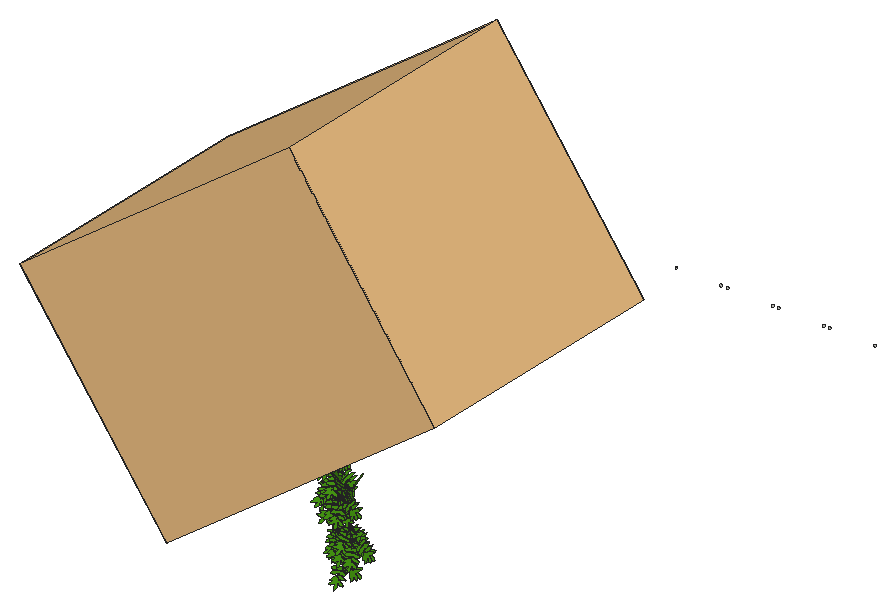
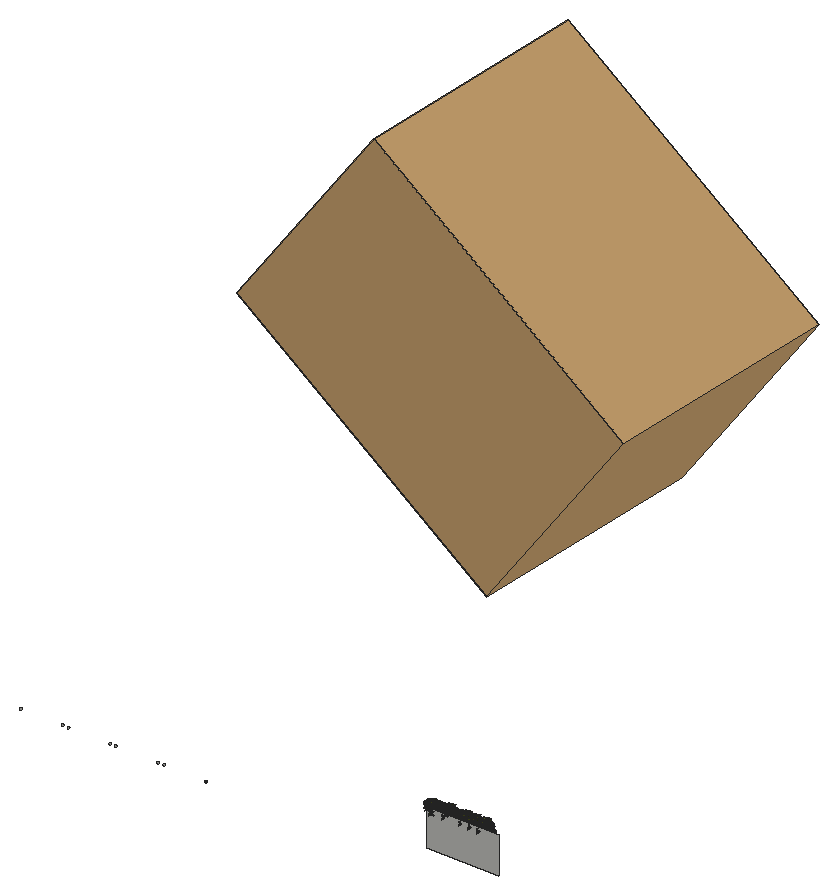
# SketchUp Ruby script. Lengths in inches.
U = 1.inch
M = Sketchup.active_model
def pt(a) = Geom::Point3d.new(a.map { |v| v * U })
def face(e, loops, mat)
  f = e.add_face(loops[0].map { |a| pt(a) })
  loops[1..].each { |l| e.add_face(l.map { |a| pt(a) }).erase! }
  f.material = f.back_material = mat if mat
  f
end
# faces: each face lists its corners as indices into pts; further lists are holes
def faces(e, pts, list, mat = nil) = list.each { |f| face(e, (f[0].is_a?(Array) ? f : [f]).map { |l| l.map { |i| pts[i] } }, mat) }
# xy, xz, yz: faces in a plane at the given z, y or x. An outline is a flat list of corners, or four numbers for a rectangle; further outlines are holes
def ring(l) = l.size == 4 ? [[l[0], l[1]], [l[2], l[1]], [l[2], l[3]], [l[0], l[3]]] : l.each_slice(2).to_a
def flat(e, list, mat, &to3) = list.each { |f| face(e, (f[0].is_a?(Array) ? f : [f]).map { |l| ring(l).map { |u, v| to3.(u, v) } }, mat) }
def xy(e, z, list, mat = nil) = flat(e, list, mat) { |x, y| [x, y, z] }
def xz(e, y, list, mat = nil) = flat(e, list, mat) { |x, z| [x, y, z] }
def yz(e, x, list, mat = nil) = flat(e, list, mat) { |y, z| [x, y, z] }
def lines(e, pts, list) = list.each { |a, b| e.add_line(pt(pts[a]), pt(pts[b])) }
# prism: a flat outline (further loops are holes) pulled along v
def prism(e, loops, v, mat = nil)
  f = face(e, loops, mat); d = Geom::Vector3d.new(v.map { |x| x * U })
  f.pushpull(f.normal.samedirection?(d) ? d.length : -d.length)
end
def box(e, o, s, mat = nil) = prism(e, [[o, [o[0] + s[0], o[1], o[2]], [o[0] + s[0], o[1] + s[1], o[2]], [o[0], o[1] + s[1], o[2]]]], [0, 0, s[2]], mat)
def at(x, y, z, deg = 0) = Geom::Transformation.translation(pt([x, y, z])) * Geom::Transformation.rotation(ORIGIN, Z_AXIS, deg.degrees)
def axes(o, x, y, z) = Geom::Transformation.new([*x, 0, *y, 0, *z, 0, *pt(o).to_a, 1])
def part(name) = M.definitions.add(name)
# library, detail: a bought-in or finely detailed component or shape, given as its bounding box
def library(name, o, s) = part(name).tap { |d| box(d.entities, o, s) }
def detail(e, o, s) = box(e.add_group.entities, o, s)
def put(e, d, t, mat = nil) = e.add_instance(d, t).tap { |i| i.material = mat if mat }
def group(e, t, mat = nil) = e.add_group.tap { |g| g.transformation = t; g.material = mat if mat }.entities
root = M.entities
M.materials.add("asdfasdfasdfasdf").color = [186, 198, 91]
M.materials.add("hojas").color = [70, 150, 19]
M.materials.add("leaf1_smaller_cleanasdfasfasdfas").color = [88, 95, 33]
M.materials.add("leaf2_smaller_cleansadfasdfasdfasd").color = [55, 66, 19]
c1 = part("rama-acacia")
p = [[-13.53,0.69,-1.07],[-13.38,0.86,-0.98],[-13.61,0.85,-1.06],[-14.07,0.85,-1.21],[-15.17,0.86,-1.58],[-15.95,0.92,-1.83],
  [-16.01,1,-1.83],[-16.01,1.17,-1.78],[-16.07,1.93,-1.6],[-16.4,2.73,-1.5],[-16.65,3.06,-1.5],[-17.13,4.01,-1.41],
  [-17.78,4.7,-1.44],[-18.28,5.07,-1.51],[-18.57,5.18,-1.58],[-18.91,5.47,-1.62],[-19.07,5.48,-1.67],[-19.35,5.61,-1.73],
  [-19.51,5.64,-1.78],[-19.38,5.57,-1.75],[-19.33,5.5,-1.75],[-19.31,5.23,-1.82],[-19.38,5.08,-1.89],[-19.41,4.84,-1.96],
  [-19.36,4.59,-2.01],[-19.43,4.55,-2.04],[-19.36,4.15,-2.125],[-19.21,3.7,-2.19],[-18.875,3.1,-2.24],[-18.61,2.78,-2.24],
  [-17.83,2.19,-2.13],[-17.4375,1.85,-2.09],[-17.04,1.49,-2.05],[-16.61,1.24,-1.97],[-16.17,1.0625,-1.87],[-16.06,0.95,-1.86],
  [-16.06,0.91,-1.87],[-16.32,0.9,-1.96],[-16.7,0.88,-2.1],[-17.05,0.91,-2.21],[-17.61,1.15,-2.33],[-18.06,1.29,-2.45],
  [-18.88,1.53,-2.67],[-20.25,1.46,-3.15],[-20.59,1.49,-3.26],[-20.79,1.37,-3.36],[-21.08,1.2,-3.5],[-21.28,1.22,-3.5625],
  [-21.48,0.94,-3.71],[-21.79,0.5,-3.93],[-22.02,0.17,-4.1],[-22.11,0.05,-4.16],[-22.21,-0.02,-4.21],[-22.375,-0.05,-4.28],
  [-22.375,-0.07,-4.28],[-22.18,-0.09,-4.22],[-22.11,-0.07,-4.19],[-21.78,-0.1,-4.09],[-21.6,-0.18,-4.05],[-21.52,-0.27,-4.04],
  [-21.33,-0.33,-4],[-20.94,-0.54,-3.92],[-20.6875,-0.63,-3.86],[-20.54,-0.68,-3.82],[-20.42,-0.67,-3.78],[-20.09,-0.46,-3.61],
  [-19.8,-0.24,-3.45],[-19.21,-0.02,-3.19],[-18.48,0.08,-2.92],[-17.72,0.38,-2.58],[-17.4,0.5,-2.4375],[-16.93,0.75,-2.21],
  [-16.78,0.8,-2.15],[-16.1,0.83,-1.91],[-16.0625,0.81,-1.9],[-16.08,0.77,-1.91],[-16.27,0.72,-1.99],[-16.88,0.39,-2.29],
  [-17.1875,0.15,-2.46],[-17.27,0.02,-2.52],[-17.94,-0.52,-2.89],[-17.94,-0.59,-2.91],[-18.08,-0.68,-2.99],[-18.13,-0.86,-3.05],
  [-18.56,-1.55,-3.38],[-18.71,-2.11,-3.58],[-18.79,-2.61,-3.74],[-18.86,-2.84,-3.83],[-18.87,-3.07,-3.89],[-18.84,-3.22,-3.92],
  [-18.8,-3.26,-3.92],[-18.76,-3.47,-3.96],[-18.76,-3.6,-4],[-18.67,-3.8,-4.02],[-18.61,-3.92,-4.04],[-18.58,-4.11,-4.07],
  [-18.53,-4.18,-4.08],[-18.58,-4.35,-4.14],[-18.65,-4.43,-4.18],[-18.72,-4.51,-4.23],[-18.8125,-4.51,-4.26],[-18.8125,-4.53,-4.26],
  [-18.72,-4.54,-4.24],[-18.66,-4.49,-4.21],[-18.58,-4.43,-4.16],[-18.35,-4.23,-4.03],[-18.32,-4.17,-4],[-18.22,-4.125,-3.95],
  [-18.1,-4,-3.88],[-17.79,-3.72,-3.7],[-17.68,-3.51,-3.61],[-17.32,-3.13,-3.38],[-17.24,-2.94,-3.31],[-16.78,-2.12,-2.93],
  [-16.48,-1.78,-2.73],[-16.3,-1.28,-2.54],[-16.05,-0.75,-2.3125],[-15.89,-0.2,-2.11],[-15.89,0.39,-1.95],[-15.96,0.79,-1.87],
  [-15.91,0.82,-1.84],[-15.27,0.8,-1.63],[-14.18,0.76,-1.27],[-13.78,0.73,-1.15],[-13.78,0.67,-1.16],[-14.23,0.54,-1.35],
  [-14.65,0.33,-1.55],[-14.97,0.02,-1.74],[-15.25,-0.36,-1.9375],[-15.57,-0.72,-2.14],[-15.96,-1.64,-2.52],[-16.2,-2.51,-2.84],
  [-16.2,-3.12,-3],[-16.14,-3.41,-3.06],[-16.1,-3.75,-3.14],[-16.1,-4.09,-3.23],[-16.2,-4.25,-3.3],[-16.2,-4.28,-3.3125],
  [-16.08,-4.19,-3.24],[-15.98,-4.08,-3.18],[-15.96,-3.94,-3.14],[-15.96,-3.8125,-3.1],[-15.9,-3.72,-3.06],[-15.68,-3.55,-2.9375],
  [-15.51,-3.49,-2.86],[-15.3,-3.33,-2.75],[-15.23,-3.17,-2.68],[-15.01,-3.03,-2.57],[-14.875,-2.83,-2.47],[-14.6,-2.59,-2.3125],
  [-14.4,-2.27,-2.16],[-14.12,-1.6,-1.89],[-13.91,-1.1,-1.68],[-13.67,-0.83,-1.53],[-13.53,-0.45,-1.38],[-13.53,0.67,-1.08],
  [-12.41,6.01,0.65],[-12.44,6.14,0.68],[-12.41,6.29,0.73],[-12.43,6.29,0.73],[-12.44,6.26,0.72],[-12.47,6.15,0.68],
  [-12.49,6.07,0.66],[-12.57,5.75,0.55],[-12.67,5.36,0.43],[-12.79,4.875,0.28],[-12.83,4.52,0.18],[-12.83,3.99,0.04],
  [-12.73,3.11,-0.18],[-12.58,2.52,-0.3125],[-12.3,1.97,-0.41],[-11.88,1.51,-0.46],[-11.37,1.0625,-0.48],[-10.75,0.75,-0.45],
  [-10.75,0.68,-0.47],[-12.55,0.7,-0.79],[-13.21,0.79,-0.89],[-13.2,0.67,-0.92],[-12.56,0.62,-0.82],[-11.15,0.56,-0.58],
  [-10.79,0.54,-0.52],[-10.72,0.52,-0.51],[-10.72,0.5,-0.52],[-10.87,0.47,-0.55],[-11.14,0.41,-0.62],[-11.39,0.27,-0.7],
  [-11.625,-0.01,-0.82],[-11.8,-0.43,-0.96],[-11.83,-0.57,-1],[-12.02,-1.08,-1.17],[-12.1,-1.39,-1.27],[-12.17,-1.95,-1.4375],
  [-12.17,-2.77,-1.65],[-12.09,-3.59,-1.86],[-11.86,-4.26,-2],[-11.8125,-4.4,-2.03],[-11.84,-4.49,-2.05],[-11.91,-4.6,-2.1],
  [-11.97,-4.65,-2.12],[-11.98,-4.67,-2.13],[-11.92,-4.65,-2.11],[-11.84,-4.59,-2.08],[-11.77,-4.52,-2.05],[-11.74,-4.47,-2.03],
  [-11.37,-4.3125,-1.92],[-10.95,-4.0625,-1.78],[-10.82,-3.89,-1.71],[-10.64,-3.57,-1.59],[-10.41,-3.05,-1.41],[-10.27,-2.73,-1.3],
  [-10.07,-1.88,-1.03],[-10.15,-0.71,-0.73],[-10.31,-0.1,-0.6],[-10.5,0.4,-0.5],[-10.5,0.48,-0.48],[-10.44,0.53,-0.45],
  [-10.39,0.64,-0.42],[-10.52,0.73,-0.42],[-10.44,0.93,-0.35],[-10.44,1.2,-0.28],[-10.32,1.47,-0.18],[-10.48,2.6875,0.12],
  [-10.43,2.96,0.2],[-10.75,3.87,0.38],[-11.26,4.93,0.57],[-11.8,5.54,0.64],[-12.37,5.93,0.64],[-7.78,0.19,-0.06],
  [-7.78,0.25,-0.04],[-7.75,0.39,0],[-7.89,0.4,-0.02],[-7.96,0.46,-0.02],[-7.96,0.49,-0.01],[-7.76,0.62,0.06],
  [-7.53,0.99,0.2],[-7.31,1.78,0.45],[-7.31,2.74,0.71],[-7.63,3.6875,0.9],[-8.02,4.57,1.07],[-8.66,5.23,1.13],
  [-8.83,5.4,1.14],[-8.92,5.54,1.16],[-9.1,5.64,1.16],[-9.08,5.6,1.15],[-9.02,5.56,1.15],[-8.94,5.46,1.14],
  [-8.9,5.37,1.12],[-8.9375,5.25,1.08],[-9.14,4.92,0.96],[-9.31,4.5625,0.83],[-9.39,3.73,0.6],[-9.44,2.76,0.32],
  [-9.23,1.59,0.05],[-8.82,0.9,-0.06],[-8.36,0.59,-0.0625],[-8.14,0.51,-0.04],[-8.05,0.48,-0.03],[-8.05,0.46,-0.04],
  [-8.12,0.43,-0.06],[-10.1,0.49,-0.4],[-8.22,0.3125,-0.11],[-8.22,0.25,-0.125],[-8.53,0.13,-0.21],[-8.8,-0.16,-0.34],
  [-8.96,-0.61,-0.49],[-8.96,-0.87,-0.56],[-9.16,-1.42,-0.74],[-9.13,-1.77,-0.83],[-9.09,-1.83,-0.84],[-9.125,-1.92,-0.87],
  [-9.125,-2.13,-0.93],[-9.08,-2.23,-0.95],[-9.15,-2.39,-1],[-9.11,-2.67,-1.07],[-9.03,-2.86,-1.11],[-9.07,-3.03,-1.16],
  [-8.97,-3.23,-1.19],[-8.93,-3.44,-1.24],[-8.93,-3.71,-1.32],[-8.79,-4.05,-1.38],[-8.7,-4.25,-1.42],[-8.7,-4.39,-1.46],
  [-8.76,-4.53,-1.5],[-8.77,-4.65,-1.54],[-8.64,-4.55,-1.49],[-8.27,-4.22,-1.33],[-8.1875,-4.06,-1.27],[-8.07,-3.98,-1.23],
  [-7.98,-3.79,-1.17],[-7.79,-3.59,-1.08],[-7.64,-3.3,-0.97],[-7.64,-3.25,-0.96],[-7.59,-3.21,-0.9375],[-7.52,-2.93,-0.85],
  [-7.52,-2.85,-0.83],[-7.47,-2.81,-0.81],[-7.3,-2.09,-0.59],[-7.32,-2.01,-0.57],[-7.27,-1.95,-0.54],[-7.1875,-1.57,-0.42],
  [-7.17,-1.46,-0.39],[-7.17,-1.16,-0.3125],[-7.23,-0.61,-0.17],[-7.49,-0.15,-0.1],[-13.39,-0.07,-1.23],[-13.39,0.25,-1.14],
  [-13.49,0.5625,-1.09],[-13.8,1.01,-1.08],[-13.61,0.91,-1.04],[-13.38,0.92,-0.96],[-13.32,1.03,-0.91],[-13.32,1.35,-0.82],
  [-13.28,1.49,-0.77],[-13.28,1.99,-0.64],[-13.44,2.67,-0.51],[-13.72,3.31,-0.43],[-13.93,3.71,-0.4],[-14.1,4.39,-0.27],
  [-14.5625,5.06,-0.25],[-14.89,5.62,-0.21],[-15.33,6.1,-0.23],[-15.65,6.8,-0.15],[-15.79,6.89,-0.18],[-15.61,6.52,-0.22],
  [-15.51,6.32,-0.24],[-15.45,6.28,-0.23],[-15.52,6,-0.32],[-15.63,5.6875,-0.45],[-15.77,4.97,-0.68],[-15.7,4.25,-0.85],
  [-15.46,3,-1.11],[-15,2.03,-1.21],[-14.3,1.29,-1.17],[-4.5625,0.33,0.09],[-4.22,0.49,0.13],[-4,0.7,0.1875],
  [-3.86,0.99,0.26],[-3.77,1.41,0.38],[-3.7,1.73,0.46],[-3.77,1.99,0.53],[-3.85,2.17,0.58],[-3.88,2.57,0.6875],
  [-3.98,2.9,0.78],[-4.0625,2.97,0.8],[-4.1,3.14,0.84],[-4.1875,3.25,0.87],[-4.27,3.55,0.95],[-4.31,3.71,0.99],
  [-4.42,3.9,1.04],[-4.625,4.2,1.125],[-4.72,4.39,1.18],[-4.89,4.57,1.23],[-4.98,4.73,1.27],[-5,4.72,1.26],
  [-5.01,4.51,1.21],[-4.96,4.32,1.16],[-4.97,4.27,1.14],[-5.14,3.78,1.01],[-5.3,3.39,0.91],[-5.44,2.76,0.74],
  [-5.5,2.09,0.56],[-5.57,1.78,0.48],[-5.57,1.42,0.38],[-5.57,1.09,0.29],[-5.47,0.72,0.19],[-5.22,0.44,0.12],
  [-4.93,0.27,0.07],[-4.76,0.22,0.06],[-4.76,0.18,0.05],[-4.83,0.16,0.04],[-5.26,0,0],[-5.34,-0.04,-0.01],
  [-5.47,-0.22,-0.06],[-5.51,-0.6,-0.16],[-5.42,-1.09,-0.29],[-5.28,-1.49,-0.4],[-5.21,-1.87,-0.5],[-5.11,-2.15,-0.57],
  [-5.08,-2.34,-0.63],[-5.01,-2.47,-0.66],[-4.96,-2.69,-0.72],[-4.86,-2.9375,-0.79],[-4.84,-3.07,-0.82],[-4.77,-3.18,-0.85],
  [-4.74,-3.43,-0.92],[-4.7,-3.71,-0.99],[-4.62,-3.89,-1.04],[-4.58,-3.98,-1.07],[-4.58,-3.83,-1.03],[-4.51,-3.67,-0.98],
  [-4.3,-3.32,-0.89],[-4.16,-3.09,-0.83],[-4.16,-2.98,-0.8],[-4.11,-2.92,-0.78],[-4.02,-2.8,-0.75],[-3.95,-2.59,-0.69],
  [-3.95,-2.33,-0.625],[-3.86,-2.26,-0.6],[-3.86,-2.02,-0.54],[-3.86,-1.44,-0.39],[-3.94,-1.22,-0.33],[-3.94,-1.08,-0.29],
  [-4,-0.96,-0.26],[-4,-0.87,-0.23],[-4.0625,-0.8125,-0.22],[-4.16,-0.54,-0.14],[-4.39,-0.24,-0.06],[-4.61,-0.08,-0.02],
  [-4.77,-0.03,-0.01],[-4.77,-0.01,0],[-4.65,-0.01,0],[-4.61,0.19,0.05],[-4.66,0.23,0.0625],[-4.63,0.29,0.08],
  [-4.07,0.17,0.04],[0,-0.24,-0.06],[0,0,0],[-0.5,0.04,0.01],[-1.58,0.08,0.02],[-13.78,0.67,-1.08]]
faces(c1.entities,p,[[0,1,2,3,4,5,6,7,8,9,10,11,12,13,14,15,16,17,18,19,20,21,22,23,24,25,26,27,28,29,30,31,32,33,34,35,36,37,38,39,40,41,42,43,44,45,46,47,48,49,50,51,52,53,54,55,56,57,58,59,60,61,62,63,64,65,66,67,68,69,70,71,72,73,74,75,76,77,78,79,80,81,82,83,84,85,86,87,88,89,90,91,92,93,94,95,96,97,98,99,100,101,102,103,104,105,106,107,108,109,110,111,112,113,114,115,116,117,118,119,120,121,122,123,124,125,126,127,128,129,130,131,132,133,134,135,136,137,138,139,140,141,142,143,144,145,146,147,148,149,150,151,152,153,154,155],[156,157,158,159,160,161,162,163,164,165,166,167,168,169,170,171,172,173,174,175,176,177,178,179,180,181,182,183,184,185,186,187,188,189,190,191,192,193,194,195,196,197,198,199,200,201,202,203,204,205,206,207,208,209,210,211,212,213,214,215,216,217,218,219,220,221,222,223,224,225,226],[227,228,229,230,231,232,233,234,235,236,237,238,239,240,241,242,243,244,245,246,247,248,249,250,251,252,253,254,255,256,257,258,216,215,259,260,261,262,263,264,265,266,267,268,269,270,271,272,273,274,275,276,277,278,279,280,281,282,283,284,285,286,287,288,289,290,291,292,293,294,295,296,297,298,299,300,301,302,303],[154,304,305,306,155],[307,308,1,309,310,311,312,313,314,315,316,317,318,319,320,321,322,323,324,325,326,327,328,329,330,331,332],[333,334,335,336,337,338,339,340,341,342,343,344,345,346,347,348,349,350,351,352,353,354,355,356,357,358,359,360,361,362,363,364,365,366,367,368,369,370,371,372,373,374,375,376,377,378,379,380,381,382,383,384,385,386,387,388,389,390,391,392,393,394,395,396,397,398,399,400,401,402,403,404,405,406,407,408,409,410,411,412,413],[0,177,1],[308,2,1],
  [176,1,177],[414,411,410,415,416,417,418],[228,370,229],[369,229,370]],"hojas")
lines(c1.entities,p,[[155,419]])
c2 = part("Group\#150")
put(c2.entities,c1,axes([10.13,10.27,0],[0.45315,0.21131,0],[-0.21131,0.45315,0],[0,0,0.5]))
put(c2.entities,c1,axes([10.13,10.27,0],[0.11638,0.47539,0.10227],[-0.48087,0.12813,-0.0484],[-0.07223,-0.08709,0.48703]))
put(c2.entities,c1,axes([9.58,10.26,-0.7],[0.1449,0.38901,-0.2787],[-0.10883,0.31035,0.37662],[0.46601,-0.04848,0.17461]))
c3 = part("Group\#151")
put(c3.entities,c2,axes([24.99,4.24,9.59],[0.78856,0.61496,0],[0.01473,-0.01889,0.99971],[0.61478,-0.78833,-0.02396]))
put(c3.entities,c2,axes([39.5,6.625,12.55],[0.6544,0.49291,0.57341],[-0.44023,-0.3682,0.81892],[0.61478,-0.78833,-0.02396]))
put(c3.entities,c2,axes([32.34,3.7,6.88],[0.78856,0.61496,0],[0.01473,-0.01889,0.99971],[0.61478,-0.78833,-0.02396]))
put(c3.entities,c2,axes([43.14,6.65,17.54],[0.78856,0.61496,0],[0.35273,-0.4523,0.81915],[0.50374,-0.64595,-0.57358]))
put(c3.entities,c2,axes([12.2,6.2,16.68],[0.7209,0.54936,0.4225],[-0.31991,-0.27701,0.90605],[0.61478,-0.78833,-0.02396]))
put(c3.entities,c2,axes([49.9375,3.79,26.09],[0.78856,0.61496,0],[0.01473,-0.01889,0.99971],[0.61478,-0.78833,-0.02396]))
put(c3.entities,c2,axes([36.11,4.9375,33.94],[0.78856,0.61496,0],[0.01473,-0.01889,0.99971],[0.61478,-0.78833,-0.02396]))
put(c3.entities,c2,axes([39.61,3.79,23.47],[0.78856,0.61496,0],[0.01473,-0.01889,0.99971],[0.61478,-0.78833,-0.02396]))
put(c3.entities,c2,axes([25.59,6.5625,46.47],[-0.40704,-0.29112,-0.86578],[0.67555,0.54201,-0.49986],[0.61478,-0.78833,-0.02396]))
put(c3.entities,c2,axes([54.97,1.98,11.65],[0.78856,0.61496,0],[0.01473,-0.01889,0.99971],[0.61478,-0.78833,-0.02396]))
put(c3.entities,c2,axes([32.97,3.79,19.14],[0.78856,0.61496,0],[0.01473,-0.01889,0.99971],[0.61478,-0.78833,-0.02396]))
put(c3.entities,c2,axes([24.24,3.79,21.99],[0.78856,0.61496,0],[0.01473,-0.01889,0.99971],[0.61478,-0.78833,-0.02396]))
put(c3.entities,c2,axes([16.86,4.24,12.3],[0.78856,0.61496,0],[0.01473,-0.01889,0.99971],[0.61478,-0.78833,-0.02396]))
put(c3.entities,c2,axes([1.23,3.9375,19.07],[0.78856,0.61496,0],[0.01473,-0.01889,0.99971],[0.61478,-0.78833,-0.02396]))
put(c3.entities,c2,axes([29.05,5.25,29.11],[0.78856,0.61496,0],[0.21033,-0.2697,0.93969],[0.57787,-0.741,-0.34202]))
put(c3.entities,c2,axes([24.16,3.79,-0.1],[0.78856,0.61496,0],[0.01473,-0.01889,0.99971],[0.61478,-0.78833,-0.02396]))
c4 = library("Sans+titre+(1)+(1)+(2)",[-30.91,-35.46,0],[63.51,67.02,85.79])
c5 = part("leaf1a")
p = [[1.06,3.74,11.78],[8.28,8.7,-0.64],[9.51,5.4,26.1],[17.76,4.04,11.26],[17.85,2.23,20],[14.31,3.29,26.73],
  [3.78,3.8125,25.98],[-0.21,2.38,19.72]]
faces(c5.entities,p,[[0,1,2],[2,1,3],[3,4,5],[3,5,2],[6,7,0],[0,2,6]],"leaf1_smaller_cleanasdfasfasdfas")
c6 = part("leaf2a")
p = [[1.4375,3.56,10.81],[8.71,6.8,-0.73],[9.51,3.5,26.59],[16.66,3.91,9.8],[17.86,1.3,19.21],[14.9,1.58,24.92],
  [5.15,2.55,24.01],[1.29,1.87,19.875]]
faces(c6.entities,p,[[0,1,2],[2,1,3],[3,4,5],[3,5,2],[6,7,0],[0,2,6]],"leaf2_smaller_cleansadfasdfasdfasd")
c7 = part("Group\#220")
put(c7.entities,c6,axes([6.68,1.92,2.42],[-0.04671,0.11082,0.08136],[0.07715,0.09226,-0.08136],[-0.11379,0.01705,-0.08856]))
put(c7.entities,c5,axes([1.26,0.54,1.25],[0.13756,-0.04533,0.01029],[0.0079,-0.00888,-0.14471],[0.04581,0.13766,-0.00594]))
put(c7.entities,c6,axes([-0.51,4.89,1.49],[-0.00057,-0.14139,-0.03304],[0.00922,0.03294,-0.14111],[0.14491,-0.00265,0.00885]))
put(c7.entities,c5,axes([4.37,7.98,1.26],[-0.14226,-0.02905,0],[0,0,-0.1452],[0.02905,-0.14226,0]))
put(c7.entities,c5,axes([1.46,4.03,4.07],[0.06242,-0.12847,-0.02614],[-0.10319,-0.03029,-0.09755],[0.08086,0.06051,-0.10432]))
c8 = part("leaf_a")
p = [[1.43,4.41,0.74],[1.39,4.36,0.69],[1.39,4.61,0.21],[1.43,4.67,0.24],[1.35,4.41,0.74],[1.35,4.67,0.24],
  [1.35,3.9,1.02],[1.43,3.9,1.02],[1.39,3.89,0.95],[1.39,3.35,0.9],[1.43,3.34,0.96],[1.35,3.34,0.96]]
faces(c8.entities,p,[[0,1,2,3],[1,4,5,2],[4,0,3,5],[3,2,5],[6,7,0,4],[8,6,4,1],[7,8,1,0],[9,10,11],
  [9,11,6,8],[10,9,8,7],[11,10,7,6]],"asdfasdfasdfasdf")
put(c8.entities,c6,axes([0,-0.08,0.875],[0.1452,0,0],[0,0.02746,-0.14258],[0,0.14258,0.02746]))
c9 = part("leaf_b")
prism(c9.entities,[[[1.36,4.21,-0.25],[1.31,4.13,-0.29],[1.26,4.21,-0.25]]],[0,-0.66,1.14],"asdfasdfasdfasdf")
put(c9.entities,c5,axes([0,-0.1,0.68],[0.1452,-0.0002,0],[0.00006,0.04124,-0.13922],[0.00019,0.13922,0.04124]))
c10 = part("Group\#209")
p = [[2.87,4.13,4.15],[2.98,3.98,4.12],[2.98,4.66,2.59],[2.87,4.8,2.65],[3.09,4.13,4.15],[3.09,4.8,2.65],
  [2.87,4.13,6.07],[2.98,3.98,6.12],[3.09,4.13,6.07],[2.87,5.04,7.34],[2.98,4.91,7.43],[3.09,5.04,7.34]]
faces(c10.entities,p,[[0,1,2,3],[1,4,5,2],[6,7,1,0],[7,8,4,1],[9,10,7,6],[10,11,8,7]],"asdfasdfasdfasdf")
put(c10.entities,c8,axes([0.86,0.51,1.53],[0.95176,-0.27809,0.12967],[0.18405,0.85554,0.48392],[-0.24551,-0.43671,0.86545]))
put(c10.entities,c9,axes([-0.97,2.96,6.52],[0.70711,-0.61237,-0.35355],[0.70711,0.61237,0.35355],[0,-0.5,0.86603]))
put(c10.entities,c8,axes([3.23,0.39,0.41],[0.82736,0.50176,-0.25242],[-0.32519,0.79434,0.5131],[0.45796,-0.34244,0.82037]))
put(c10.entities,c8,axes([3.25,-0.58,4.78],[0.8251,0.44069,-0.35355],[-0.31829,0.8796,0.35355],[0.46679,-0.17918,0.86603]))
c11 = part("Group\#2")
p = [[1.22,4.71,2.14],[1.31,4.57,2.14],[2.16,4.71,3.79],[2.24,4.57,3.77],[1.39,4.71,2.14],[2.33,4.71,3.79],
  [1.93,3.51,6.2],[1.85,3.64,6.23],[2.02,3.64,6.23],[0.93,3.38,8.58],[0.85,3.52,8.58],[1.02,3.52,8.58],
  [0.81,3.57,10.77],[0.72,3.71,10.73],[0.89,3.71,10.73],[1.31,4.57,13.2],[1.22,4.7,13.15],[1.39,4.7,13.15]]
faces(c11.entities,p,[[0,1,2],[3,2,1],[1,4,3],[5,3,4],[6,7,3],[6,3,8],[2,3,7],[5,8,3],
  [9,10,6],[9,6,11],[7,6,10],[8,11,6],[9,11,12],[9,12,10],[13,10,12],[14,12,11],
  [12,15,13],[12,14,15],[16,13,15],[17,15,14]],"asdfasdfasdfasdf")
put(c11.entities,c9,axes([3.93,1.17,1.97],[0.75139,0.49793,0.43299],[-0.65983,0.56085,0.50006],[0.00615,-0.66145,0.74997]))
put(c11.entities,c9,axes([6.23,5.09,1.92],[-0.36585,0.92196,0.12706],[-0.79398,-0.38042,0.47421],[0.48554,0.0726,0.87119]))
put(c11.entities,c9,axes([0.03,0.92,11.26],[1,0,0],[0,0.86603,0.5],[0,-0.5,0.86603]))
put(c11.entities,c8,axes([4.37,2.0625,9.11],[0.45529,0.76896,0.44879],[-0.86129,0.25267,0.44084],[0.22559,-0.58725,0.77733]))
put(c11.entities,c8,axes([1.89,-0.25,4.42],[0.88717,0.14116,0.43931],[-0.36372,0.79981,0.47751],[-0.28396,-0.58342,0.76091]))
put(c11.entities,c8,axes([-0.4,-0.0625,7.9],[0.80178,0.42258,-0.42258],[0,0.70711,0.70711],[0.59763,-0.56694,0.56694]))
put(c11.entities,c9,axes([0.05,0.6875,0.65],[0.97178,0.10445,-0.21151],[0.0126,0.87237,0.48869],[0.23556,-0.47756,0.84643]))
put(c11.entities,c8,axes([5.56,1.19,4.08],[0.24789,0.96746,-0.05068],[-0.86286,0.24427,0.4425],[0.44048,-0.06596,0.89533]))
put(c11.entities,c9,axes([4.91,2.14,7.29],[-0.04249,0.96546,-0.25705],[-0.89911,0.07524,0.4312],[0.43565,0.24944,0.86486]))
c12 = part("Group\#208")
put(c12.entities,c6,axes([5.59,5.52,3.3],[-0.07606,0.12201,-0.02028],[0.09645,0.0436,-0.0994],[-0.07744,-0.06554,-0.10388]))
put(c12.entities,c6,axes([7.69,4.27,1.08],[-0.09839,0.10661,0.00609],[-0.00698,0.00184,-0.14502],[-0.10656,-0.09856,0.00388]))
put(c12.entities,c5,axes([3.51,6.9,2.1],[-0.1403,-0.03711,-0.00465],[-0.00046,0.01976,-0.14385],[0.03739,-0.13898,-0.01921]))
put(c12.entities,c6,axes([2.18,0.07,1.375],[0.14025,0.00096,-0.03757],[-0.03758,0.00358,-0.14021],[0,0.14515,0.00371]))
put(c12.entities,c5,axes([-0.62,2,1.16],[0.081,-0.0806,-0.00996],[0.00004,0.01411,-0.11384],[0.08122,0.08039,0.00999]))
c13 = part("Group\#221")
p = [[1.22,4.71,2.14],[1.31,4.57,2.14],[2.16,4.71,3.79],[2.24,4.57,3.77],[1.39,4.71,2.14],[2.33,4.71,3.79],
  [1.93,3.51,6.2],[1.85,3.64,6.23],[2.02,3.64,6.23],[0.93,3.38,8.58],[0.85,3.52,8.58],[1.02,3.52,8.58],
  [0.81,3.57,10.77],[0.72,3.71,10.73],[0.89,3.71,10.73],[1.31,4.57,13.2],[1.22,4.7,13.15],[1.39,4.7,13.15]]
faces(c13.entities,p,[[0,1,2],[3,2,1],[1,4,3],[5,3,4],[6,7,3],[6,3,8],[2,3,7],[5,8,3],
  [9,10,6],[9,6,11],[7,6,10],[8,11,6],[9,11,12],[9,12,10],[13,10,12],[14,12,11],
  [12,15,13],[12,14,15],[16,13,15],[17,15,14]],"asdfasdfasdfasdf")
put(c13.entities,c9,axes([3.93,1.17,1.97],[0.75139,0.49793,0.43299],[-0.65983,0.56085,0.50006],[0.00615,-0.66145,0.74997]))
put(c13.entities,c9,axes([6.23,5.09,1.92],[-0.36585,0.92196,0.12706],[-0.79398,-0.38042,0.47421],[0.48554,0.0726,0.87119]))
put(c13.entities,c9,axes([0.03,0.92,11.26],[1,0,0],[0,0.86603,0.5],[0,-0.5,0.86603]))
put(c13.entities,c8,axes([4.37,2.0625,9.11],[0.45529,0.76896,0.44879],[-0.86129,0.25267,0.44084],[0.22559,-0.58725,0.77733]))
put(c13.entities,c8,axes([1.89,-0.25,4.42],[0.88717,0.14116,0.43931],[-0.36372,0.79981,0.47751],[-0.28396,-0.58342,0.76091]))
put(c13.entities,c8,axes([-0.4,-0.0625,7.9],[0.80178,0.42258,-0.42258],[0,0.70711,0.70711],[0.59763,-0.56694,0.56694]))
put(c13.entities,c9,axes([0.05,0.6875,0.65],[0.97178,0.10445,-0.21151],[0.0126,0.87237,0.48869],[0.23556,-0.47756,0.84643]))
put(c13.entities,c8,axes([5.56,1.19,4.08],[0.24789,0.96746,-0.05068],[-0.86286,0.24427,0.4425],[0.44048,-0.06596,0.89533]))
put(c13.entities,c9,axes([4.91,2.14,7.29],[-0.04249,0.96546,-0.25705],[-0.89911,0.07524,0.4312],[0.43565,0.24944,0.86486]))
c14 = part("Trailing philodendron")
put(c14.entities,c5,axes([3.65,12.52,19.68],[-0.0527,-0.13492,0.0101],[-0.03487,0.00307,-0.14092],[0.13073,-0.05357,-0.03351]))
put(c14.entities,c5,axes([5.13,11.34,20.6],[-0.03432,-0.12484,0.06572],[-0.08608,-0.03507,-0.11155],[0.11179,-0.06533,-0.06572]))
put(c14.entities,c6,axes([2.61,13.04,18.63],[0.05838,-0.12752,0.03758],[0.01564,-0.03417,-0.14025],[0.13202,0.06044,0]))
put(c14.entities,c6,axes([3.7,9.83,20.73],[-0.00129,-0.14519,0],[-0.0726,0.00064,-0.12575],[0.12574,-0.00112,-0.0726]))
put(c14.entities,c6,axes([11.375,11.11,20.23],[-0.14171,0.00126,0.03163],[-0.02867,0.05638,-0.1307],[-0.01341,-0.1338,-0.05478]))
put(c14.entities,c5,axes([2.4375,12.45,15.12],[-0.02375,-0.14324,0],[0.13106,-0.02173,-0.05859],[0.05781,-0.00958,0.13285]))
put(c14.entities,c5,axes([9.62,10.68,22.01],[0.05693,0.12487,-0.04742],[0.05061,-0.06787,-0.11796],[-0.12361,0.02972,-0.07014]))
put(c14.entities,c5,axes([11.63,16.35,20.5625],[-0.12691,-0.00762,0.07014],[-0.06947,0.03872,-0.12148],[-0.01233,-0.13973,-0.03749]))
put(c14.entities,c5,axes([12.51,17.52,17.81],[-0.1445,0.01001,0.0102],[-0.01383,-0.07182,-0.12544],[-0.0036,-0.1258,0.07242]))
put(c14.entities,c6,axes([9.09,6.34,22.72],[-0.09269,-0.05068,-0.09962],[-0.03661,0.13604,-0.03515],[0.1056,0.00268,-0.09962]))
put(c14.entities,c5,axes([4.83,12.62,22.54],[0.10783,0.09684,-0.00888],[0.09716,-0.10783,0.00397],[-0.00394,-0.00889,-0.14487]))
put(c14.entities,c5,axes([4.94,9.48,20.375],[0.01323,0.07633,0.07653],[0.10803,-0.00667,-0.01203],[-0.00375,0.07738,-0.07653]))
put(c14.entities,c6,axes([14,13.64,21.84],[-0.01852,-0.13907,0.03741],[-0.14373,0.01547,-0.01367],[0.00911,-0.03878,-0.13963]))
put(c14.entities,c6,axes([9.23,4.15,18.71],[0.14198,0.00177,-0.03038],[-0.02867,0.05638,-0.1307],[0.01021,0.13379,0.05548]))
put(c14.entities,c6,axes([5.82,4.5625,15.3],[0.13095,-0.05433,0.03137],[0.06268,0.11013,-0.07089],[0.00273,0.07747,0.12278]))
put(c14.entities,c7,axes([6.59,5.29,16.06],[1.23201,0.26412,0],[-0.26412,1.23201,0],[0,0,1.26]))
put(c14.entities,c10,axes([12.21,1.69,0.66],[-0.82914,0.03045,-0.02227],[0.02366,0.80139,0.21474],[-0.02938,-0.21389,0.80143]))
put(c14.entities,c11,axes([6.8125,1.15,7.57],[0.74375,-0.41052,0.02847],[0.41052,0.73612,-0.11],[0.02847,0.11,0.84237]))
put(c14.entities,c10,axes([-1.68,6.875,13.2],[0.5,-0.86603,0],[0.81585,0.47103,-0.33545],[0.29051,0.16773,0.94206]))
put(c14.entities,c10,axes([1.86,19.56,12.8125],[0.88164,0.4704,0.03781],[0.46333,-0.8476,-0.25863],[0.08962,-0.24554,0.96524]))
g1 = group(c14.entities,at(9.13,11.13,20.67))
put(g1,c6,axes([7.36,4.03,-0.3],[-0.05057,0.11966,-0.06487],[0.07036,-0.03625,-0.12173],[-0.11651,-0.07383,-0.04536]))
put(g1,c6,axes([8.4,1.56,-2.35],[-0.06703,0.12496,-0.03122],[-0.04831,-0.05702,-0.12449],[-0.1194,-0.04708,0.0679]))
put(g1,c5,axes([5.37,5.58,-2.1],[-0.14013,0.0124,0.03596],[-0.03803,-0.04347,-0.13322],[-0.00061,-0.13798,0.0452]))
put(g1,c6,axes([2.45,-0.07,0.8],[0.12002,-0.06072,-0.05468],[-0.07506,-0.04353,-0.11642],[0.03229,0.1245,-0.06737]))
put(g1,c5,axes([0.19,2.38,0.125],[0.05529,-0.09889,0.01797],[-0.03005,-0.03583,-0.10474],[0.09591,0.04578,-0.04318]))
put(c14.entities,c12,axes([17.33,10.54,16.15],[-0.62797,0.46654,0.62289],[-0.59637,-0.80271,0],[0.5,-0.37147,0.78231]))
put(c14.entities,c7,axes([3.44,11.88,17.73],[0.78616,-0.36326,0.5],[0.52263,0.82256,-0.22414],[-0.32986,0.43753,0.83652]))
put(c14.entities,c12,axes([5.5,5.07,16.54],[0.96593,-0.11102,0.2338],[0,0.90334,0.42894],[-0.25882,-0.41432,0.87255]))
put(c14.entities,c10,axes([18.84,3.62,12.91],[-0.80696,-0.59061,0],[-0.57048,0.77946,-0.25882],[-0.15286,0.20886,0.96593]))
put(c14.entities,c11,axes([3.89,0.96,5.21],[0.83948,0.00528,-0.02906],[-0.009,0.83292,-0.10846],[0.02813,0.1087,0.83246]))
put(c14.entities,c11,axes([6.1,0.84,-5.33],[0.875,-0.48296,0.03349],[0.48296,0.86603,-0.12941],[0.03349,0.12941,0.99103]))
put(c14.entities,c11,axes([3.87,-0.55,-8.84],[0.99938,0.00629,-0.0346],[-0.01071,0.99157,-0.12912],[0.03349,0.12941,0.99103]))
put(c14.entities,c10,axes([0.46,6.875,13.01],[0.5,-0.86603,0],[0.81585,0.47103,-0.33545],[0.29051,0.16773,0.94206]))
put(c14.entities,c11,axes([10.39,0.84,1.73],[0.875,-0.48296,0.03349],[0.48296,0.86603,-0.12941],[0.03349,0.12941,0.99103]))
put(c14.entities,c11,axes([-0.75,1.13,2.67],[0.7525,-0.41535,0.0288],[0.41535,0.74478,-0.11129],[0.0288,0.11129,0.85228]))
put(c14.entities,c11,axes([0.04,-0.97,-8.67],[0.735,-0.40569,0.02813],[0.40569,0.72746,-0.1087],[0.02813,0.1087,0.83246]))
put(c14.entities,c11,axes([0.09,-0.6,-7.42],[0.47403,-0.32078,-0.33698],[0.20171,0.57521,-0.26383],[0.41925,0.08595,0.50794]))
put(c14.entities,c11,axes([10.35,0.97,-6.0625],[0.76125,-0.42018,0.02914],[0.42018,0.75344,-0.11259],[0.02914,0.11259,0.86219]))
put(c14.entities,c11,axes([10.78,-1.55,-11.77],[0.72777,-0.42018,0.22517],[0.435,0.75344,0],[-0.19501,0.11259,0.84036]))
put(c14.entities,c11,axes([5.78,-1.55,-20.23],[0.76125,-0.42018,0.02914],[0.42018,0.75344,-0.11259],[0.02914,0.11259,0.86219]))
put(c14.entities,c11,axes([8.72,-1.43,-13.97],[0.65467,-0.36135,0.02506],[0.36135,0.64796,-0.09682],[0.02506,0.09682,0.74149]))
put(c14.entities,c13,axes([1.53,-0.97,-19.86],[0.735,-0.40569,0.02813],[0.40569,0.72746,-0.1087],[0.02813,0.1087,0.83246]))
put(c14.entities,c13,axes([6.23,-2.02,-7.18],[0.55125,-0.30427,0.0211],[0.39555,0.70927,-0.10599],[0.0211,0.08153,0.62435]))
put(c14.entities,c13,axes([6.43,-1.89,6.18],[0.735,-0.40569,0.02813],[0.5274,0.9457,-0.14132],[0.02813,0.1087,0.83246]))
put(c14.entities,c13,axes([10.24,1.09,9.64],[0.62475,-0.34484,0.02391],[0.44829,0.80384,-0.12012],[0.02391,0.0924,0.70759]))
put(c14.entities,c10,axes([1.56,7.74,12.8125],[-0.22619,0.97335,0.03781],[0.93864,0.22817,-0.25863],[0.26037,0.02301,0.96524]))
put(c14.entities,c10,axes([0.65,14.36,12.8125],[0.30411,0.95189,0.03781],[0.92309,-0.28464,-0.25863],[0.23543,-0.11355,0.96524]))
put(c14.entities,c10,axes([7.75,10.38,12.8125],[-0.84074,0.54011,0.03781],[0.51385,0.81797,-0.25863],[0.17062,0.19802,0.96524]))
put(c14.entities,c10,axes([12.92,19.16,12.8125],[0.9234,-0.38197,0.03781],[-0.36017,-0.89632,-0.25863],[-0.13268,-0.22521,0.96524]))
put(c14.entities,c10,axes([6.55,17.22,12.8125],[0.7985,0.60081,0.03781],[0.58857,-0.76596,-0.25863],[0.12643,-0.22877,0.96524]))
put(c14.entities,c10,axes([16.24,8.94,12.8125],[-0.64953,-0.75939,0.03781],[-0.7404,0.62041,-0.25863],[-0.17295,0.19599,0.96524]))
put(c14.entities,c10,axes([15.6875,15.74,12.8125],[0.12972,-0.99083,0.03781],[-0.95648,-0.13509,-0.25863],[-0.26137,0.00261,0.96524]))
put(c14.entities,c10,axes([19.85,8,15.61],[-0.64953,-0.75939,0.03781],[-0.7404,0.62041,-0.25863],[-0.17295,0.19599,0.96524]))
put(c14.entities,c10,axes([18.86,17.5,12.8125],[0.62831,-0.77705,0.03781],[-0.74495,-0.61494,-0.25863],[-0.22422,-0.13434,0.96524]))
put(c14.entities,c10,axes([-0.43,13.28,13.2],[-0.41945,-0.90778,0],[0.85518,-0.39515,-0.33545],[0.30452,-0.14071,0.94206]))
put(c14.entities,c13,axes([4.5625,-2.01,7.45],[0.56595,-0.31238,0.02166],[0.40609,0.72819,-0.10881],[0.02166,0.0837,0.641]))
put(c14.entities,c13,axes([4.48,-2.02,-24.24],[0.55125,-0.30427,0.0211],[0.39555,0.70927,-0.10599],[0.0211,0.08153,0.62435]))
put(c14.entities,c13,axes([4.9,-4.23,-11.04],[0.55125,-0.30427,0.0211],[0.39555,0.70927,-0.10599],[0.0211,0.08153,0.62435]))
put(c14.entities,c12,axes([17.33,10.54,17.41],[-0.62797,0.46654,0.62289],[-0.59637,-0.80271,0],[0.5,-0.37147,0.78231]))
put(c14.entities,c10,axes([-0.03,6.82,20.63],[0.44714,-0.87214,-0.19857],[0.53417,0.43844,-0.7228],[0.71744,0.21712,0.66191]))
put(c14.entities,c10,axes([20.82,12.8,12.8125],[0.12972,-0.99083,0.03781],[-0.95648,-0.13509,-0.25863],[-0.26137,0.00261,0.96524]))
xz(root,776.37,[[2273.89,138.1875,2360.78,183.3125]])
xz(root,799.91,[[2612.5,131.88,2612.79,131.92,2613.06,132.03,2613.29,132.21,2613.47,132.44,2613.58,132.71,2613.62,133,2613.58,133.29,2613.47,133.57,2613.29,133.8,2613.06,133.98,2612.79,134.09,2612.5,134.13,2612.21,134.09,2611.93,133.98,2611.7,133.8,2611.52,133.57,2611.41,133.29,2611.37,133,2611.41,132.71,2611.52,132.44,2611.7,132.21,2611.93,132.03,2612.21,131.92],[2663.62,131.88,2663.91,131.92,2664.18,132.03,2664.42,132.21,2664.6,132.44,2664.71,132.71,2664.75,133,2664.71,133.29,2664.6,133.57,2664.42,133.8,2664.18,133.98,2663.91,134.09,2663.62,134.13,2663.33,134.09,2663.06,133.98,2662.83,133.8,2662.65,133.57,2662.53,133.29,2662.5,133,2662.53,132.71,2662.65,132.44,2662.83,132.21,2663.06,132.03,2663.33,131.92],[2671.48,131.88,2671.78,131.92,2672.05,132.03,2672.28,132.21,2672.46,132.44,2672.57,132.71,2672.61,133,2672.57,133.29,2672.46,133.57,2672.28,133.8,2672.05,133.98,2671.78,134.09,2671.48,134.13,2671.19,134.09,2670.92,133.98,2670.6875,133.8,2670.51,133.57,2670.4,133.29,2670.36,133,2670.4,132.71,2670.51,132.44,2670.6875,132.21,2670.92,132.03,2671.19,131.92],[2722.61,131.88,2722.9,131.92,2723.17,132.03,2723.41,132.21,2723.58,132.44,2723.7,132.71,2723.73,133,2723.7,133.29,2723.58,133.57,2723.41,133.8,2723.17,133.98,2722.9,134.09,2722.61,134.13,2722.32,134.09,2722.05,133.98,2721.8125,133.8,2721.64,133.57,2721.52,133.29,2721.48,133,2721.52,132.71,2721.64,132.44,2721.8125,132.21,2722.05,132.03,2722.32,131.92],[2729.66,131.88,2729.95,131.92,2730.22,132.03,2730.46,132.21,2730.63,132.44,2730.75,132.71,2730.79,133,2730.75,133.29,2730.63,133.57,2730.46,133.8,2730.22,133.98,2729.95,134.09,2729.66,134.13,2729.37,134.09,2729.1,133.98,2728.86,133.8,2728.6875,133.57,2728.57,133.29,2728.54,133,2728.57,132.71,2728.6875,132.44,2728.86,132.21,2729.1,132.03,2729.37,131.92],
  [2780.79,131.88,2781.08,131.92,2781.35,132.03,2781.58,132.21,2781.76,132.44,2781.87,132.71,2781.91,133,2781.87,133.29,2781.76,133.57,2781.58,133.8,2781.35,133.98,2781.08,134.09,2780.79,134.13,2780.49,134.09,2780.22,133.98,2779.99,133.8,2779.8125,133.57,2779.7,133.29,2779.66,133,2779.7,132.71,2779.8125,132.44,2779.99,132.21,2780.22,132.03,2780.49,131.92],[2787.96,131.88,2788.25,131.92,2788.52,132.03,2788.76,132.21,2788.94,132.44,2789.05,132.71,2789.09,133,2789.05,133.29,2788.94,133.57,2788.76,133.8,2788.52,133.98,2788.25,134.09,2787.96,134.13,2787.67,134.09,2787.4,133.98,2787.17,133.8,2786.99,133.57,2786.875,133.29,2786.84,133,2786.875,132.71,2786.99,132.44,2787.17,132.21,2787.4,132.03,2787.67,131.92],[2839.09,131.88,2839.38,131.92,2839.65,132.03,2839.88,132.21,2840.06,132.44,2840.17,132.71,2840.21,133,2840.17,133.29,2840.06,133.57,2839.88,133.8,2839.65,133.98,2839.38,134.09,2839.09,134.13,2838.8,134.09,2838.52,133.98,2838.29,133.8,2838.11,133.57,2838,133.29,2837.96,133,2838,132.71,2838.11,132.44,2838.29,132.21,2838.52,132.03,2838.8,131.92]])
p = [[2611.37,801.78,133],[2611.41,801.78,132.71],[2611.41,799.91,132.71],[2611.37,799.91,133],[2611.41,801.78,133.29],[2611.41,799.91,133.29]]
faces(root,p,[[0,1,2,3],[4,0,3,5]])
put(root,c3,axes([2840.12,103.66,150.12],[-2.13366,1.79036,0],[-1.79036,-2.13366,0],[0,0,2.7853]))
put(root,c4,axes([2823.86,247.05,494.92],[-2.63478,0,3.57373],[0,4.44,0],[-3.57373,0,-2.63478]))
put(root,c14,axes([2290.02,757.41,163.27],[1.02772,-0.11891,0],[0.11891,1.02772,0],[0,0,1.03457]))
put(root,c14,axes([2333.27,757.41,163.27],[1.02772,-0.11891,0],[0.11891,1.02772,0],[0,0,1.03457]))
put(root,c14,axes([2312.57,757.84,163.85],[1.00674,-0.11648,0],[0.11648,1.00674,0],[0,0,1.01346]))
put(root,c14,axes([2301.24,758.42,164.63],[0.97878,-0.11325,0],[0.11325,0.97878,0],[0,0,0.98531]))
put(root,c14,axes([2348.24,760.14,164.61],[0.94382,-0.1092,0],[0.1092,0.94382,0],[0,0,0.95012]))
put(root,c14,axes([2331.6875,764.1875,172.43],[0.69913,-0.08089,0],[0.08089,0.69913,0],[0,0,0.70379]))
put(root,c14,axes([2352.9375,764.1875,172.43],[0.69913,-0.08089,0],[0.08089,0.69913,0],[0,0,0.70379]))
